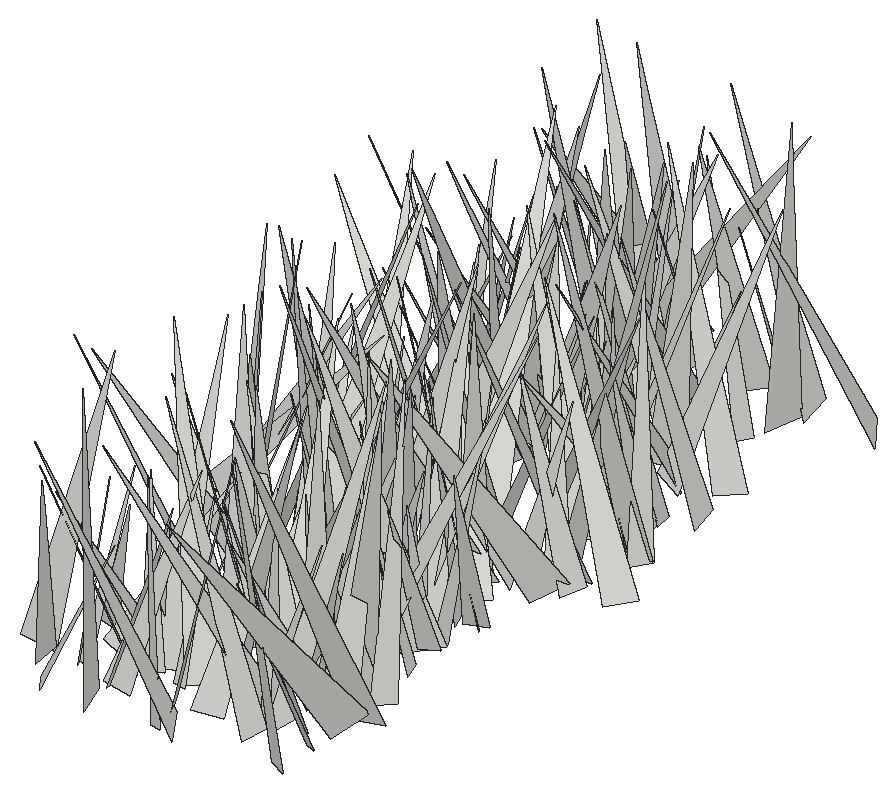
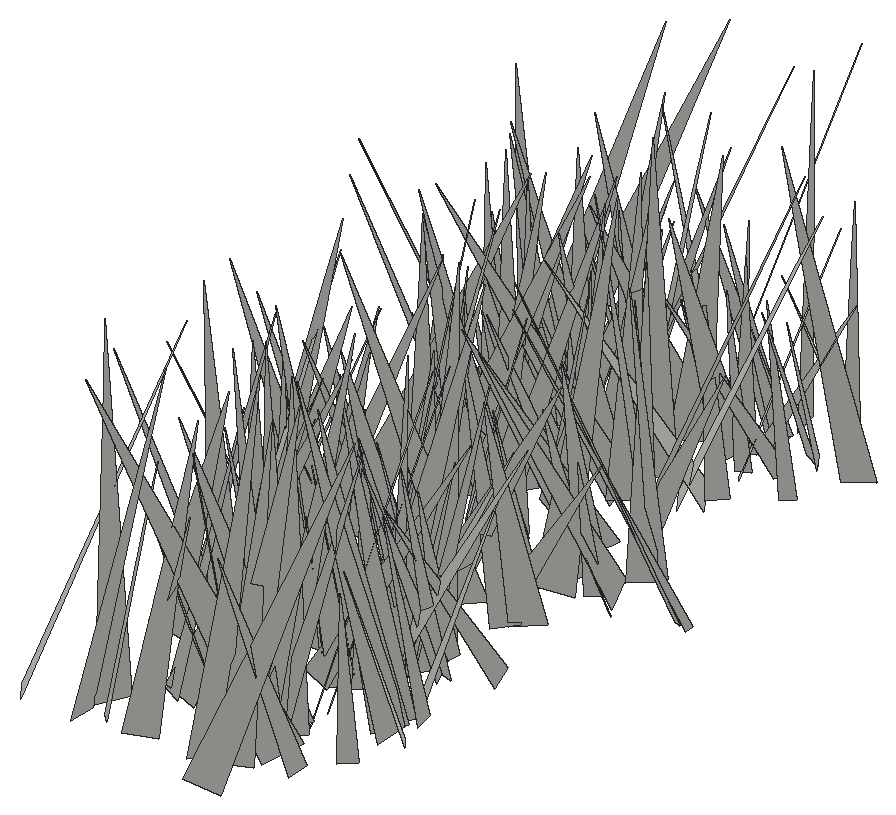
# SketchUp Ruby script. Lengths in inches.
U = 1.inch
M = Sketchup.active_model
def pt(a) = Geom::Point3d.new(a.map { |v| v * U })
def face(e, loops, mat)
  f = e.add_face(loops[0].map { |a| pt(a) })
  loops[1..].each { |l| e.add_face(l.map { |a| pt(a) }).erase! }
  f.material = f.back_material = mat if mat
  f
end
# faces: each face lists its corners as indices into pts; further lists are holes
def faces(e, pts, list, mat = nil) = list.each { |f| face(e, (f[0].is_a?(Array) ? f : [f]).map { |l| l.map { |i| pts[i] } }, mat) }
# xy, xz, yz: faces in a plane at the given z, y or x. An outline is a flat list of corners, or four numbers for a rectangle; further outlines are holes
def ring(l) = l.size == 4 ? [[l[0], l[1]], [l[2], l[1]], [l[2], l[3]], [l[0], l[3]]] : l.each_slice(2).to_a
def flat(e, list, mat, &to3) = list.each { |f| face(e, (f[0].is_a?(Array) ? f : [f]).map { |l| ring(l).map { |u, v| to3.(u, v) } }, mat) }
def xy(e, z, list, mat = nil) = flat(e, list, mat) { |x, y| [x, y, z] }
def xz(e, y, list, mat = nil) = flat(e, list, mat) { |x, z| [x, y, z] }
def yz(e, x, list, mat = nil) = flat(e, list, mat) { |y, z| [x, y, z] }
def lines(e, pts, list) = list.each { |a, b| e.add_line(pt(pts[a]), pt(pts[b])) }
# prism: a flat outline (further loops are holes) pulled along v
def prism(e, loops, v, mat = nil)
  f = face(e, loops, mat); d = Geom::Vector3d.new(v.map { |x| x * U })
  f.pushpull(f.normal.samedirection?(d) ? d.length : -d.length)
end
def box(e, o, s, mat = nil) = prism(e, [[o, [o[0] + s[0], o[1], o[2]], [o[0] + s[0], o[1] + s[1], o[2]], [o[0], o[1] + s[1], o[2]]]], [0, 0, s[2]], mat)
def at(x, y, z, deg = 0) = Geom::Transformation.translation(pt([x, y, z])) * Geom::Transformation.rotation(ORIGIN, Z_AXIS, deg.degrees)
def axes(o, x, y, z) = Geom::Transformation.new([*x, 0, *y, 0, *z, 0, *pt(o).to_a, 1])
def part(name) = M.definitions.add(name)
# library, detail: a bought-in or finely detailed component or shape, given as its bounding box
def library(name, o, s) = part(name).tap { |d| box(d.entities, o, s) }
def detail(e, o, s) = box(e.add_group.entities, o, s)
def put(e, d, t, mat = nil) = e.add_instance(d, t).tap { |i| i.material = mat if mat }
def group(e, t, mat = nil) = e.add_group.tap { |g| g.transformation = t; g.material = mat if mat }.entities
root = M.entities
c1 = part("fur_instance\#9")
p = [[0.8125,0,1.79],[0.67,-0.02,1.48],[0,-0.11,0],[0,0.11,0]]
faces(c1.entities,p,[[0,1,2,3]])
put(root,c1,axes([142.74,11.99,-27.1],[-6.5639,-4.29471,0.69968],[-4.06333,6.50273,1.7952],[1.55674,-1.13527,7.63588]))
put(root,c1,axes([138.88,11.62,-27.1],[6.72646,1.81373,2.96578],[2.30607,-7.16166,-0.85049],[-2.60144,-1.65881,6.91459]))
put(root,c1,axes([148.02,16.27,-27.1],[5.96387,-5.74764,0.45925],[-4.68382,-5.21453,-4.43673],[-3.36276,-2.93042,6.99418]))
put(root,c1,axes([135.31,13.3,-27.1],[5.21183,-0.69159,1.00189],[-0.40075,-5.13378,-1.45906],[-1.14955,-1.3458,5.051]))
put(root,c1,axes([136.49,11.45,-27.1],[3.11612,2.14822,0.04863],[2.13222,-3.08072,-0.53874],[0.26618,-0.47091,3.74631]))
put(root,c1,axes([147.85,11.98,-27.1],[-3.61019,-4.99925,2.09321],[-5.40705,3.49453,-0.97958],[0.37125,2.28107,6.08822]))
put(root,c1,axes([144.81,15.47,-27.1],[-6.99156,-3.62516,0.34789],[-3.32905,6.6672,2.57109],[1.47657,-2.13338,7.444]))
put(root,c1,axes([142.17,11.5,-27.1],[2.11114,4.26728,1.69749],[4.08085,-2.60007,1.46097],[-2.10662,-0.76029,4.53125]))
put(root,c1,axes([141.64,13.32,-27.1],[5.91305,2.63208,1.30513],[2.84881,-5.85376,-1.10147],[-0.71801,-1.54954,6.37799]))
put(root,c1,axes([147.875,14,-27.1],[-2.11494,-3.26023,0.3236],[-3.25153,2.04149,-0.68318],[-0.40176,0.64034,3.82562]))
put(root,c1,axes([138.71,13.3,-27.1],[4.6292,0.17151,0.50537],[0.17521,-4.6565,-0.02456],[-0.5041,-0.0434,4.63231]))
put(root,c1,axes([139.07,12.98,-27.1],[-0.2633,5.21725,2.01289],[5.21535,0.95622,-1.79623],[2.01778,-1.79073,4.90536]))
put(root,c1,axes([145.59,13.39,-27.1],[-7.05219,-0.0174,0.36445],[-0.04272,7.04446,-0.49029],[0.36236,0.49184,7.03515]))
put(root,c1,axes([138.22,16.61,-27.1],[-4.13321,-3.41194,0.20507],[-3.07913,3.85633,2.10107],[1.48403,-1.5014,4.93054]))
put(root,c1,axes([148.3125,16.93,-27.1],[0.33917,-8.30019,0.61155],[-8.21231,-0.43312,-1.32383],[-1.35096,0.54903,8.20095]))
put(root,c1,axes([138.89,14.33,-27.1],[-3.23089,-3.2407,0.20186],[-3.09319,2.98531,-1.58167],[-0.98745,1.25194,4.29408]))
put(root,c1,axes([134.44,13.88,-27.1],[1.86303,-6.4471,2.90273],[-6.99316,-1.23765,1.73947],[1.04242,3.21946,6.48153]))
put(root,c1,axes([146.71,14.99,-27.1],[-2.94659,-4.28728,0.79485],[-4.35538,2.84813,-0.78348],[-0.2081,1.09651,5.14289]))
put(root,c1,axes([136.61,13.6875,-27.1],[2.93854,2.24557,1.05284],[2.03507,-3.11619,0.96641],[-1.41759,0.18132,3.56983]))
put(root,c1,axes([145.97,14.85,-27.1],[-4.77809,0.40303,0.49366],[0.4272,4.79644,0.21897],[0.47289,-0.2608,4.79006]))
put(root,c1,axes([145.02,14.45,-27.1],[2.48119,3.58815,0.88423],[3.68479,-2.32113,-0.92071],[0.2811,-1.24521,4.2642]))
put(root,c1,axes([146.04,16.8,-27.1],[2.95419,-3.46444,1.08183],[-2.95275,-3.10527,-1.88109],[-2.11044,-0.50488,4.14621]))
put(root,c1,axes([139.31,14.87,-27.1],[1.67153,-3.68103,1.97281],[-4.08391,-1.88531,-0.05752],[-0.87388,1.76964,4.04237]))
put(root,c1,axes([136.89,13.69,-27.1],[1.45638,3.8911,0.37542],[3.87774,-1.48869,0.38679],[-0.49475,-0.21394,4.13668]))
put(root,c1,axes([138.44,16.03,-27.1],[0.50859,-3.54434,0.97529],[-3.61365,-0.30136,0.78924],[0.67458,1.05784,3.49258]))
put(root,c1,axes([135.71,16.69,-27.1],[0.50493,-3.90237,0.56248],[-3.75126,-0.30094,1.27958],[1.21364,0.69337,3.72104]))
put(root,c1,axes([142.125,16.17,-27.1],[6.74375,-1.56753,0.95704],[-1.61805,-6.79399,0.27364],[-0.86892,0.48558,6.91813]))
put(root,c1,axes([140.84,14.64,-27.1],[1.32341,3.79294,0.4756],[3.74321,-1.38791,0.65276],[-0.77522,-0.22654,3.9638]))
put(root,c1,axes([142.03,18.27,-27.1],[-4.79038,-5.44103,1.36632],[-5.2062,4.98101,1.5825],[2.08977,-0.06337,7.07448]))
put(root,c1,axes([144,16.3,-27.1],[0.99186,4.25892,2.03749],[4.71935,-0.95274,-0.30591],[-0.13232,-2.05608,4.36218]))
put(root,c1,axes([141.59,15.37,-27.1],[-4.74257,5.72398,1.5327],[5.90767,4.72004,0.65254],[0.46105,-1.60076,7.40474]))
put(root,c1,axes([143.11,13.57,-27.1],[-4.70627,4.28235,1.06672],[3.70191,4.67966,-2.45399],[2.40255,1.178,5.87073]))
put(root,c1,axes([136.97,15.39,-27.1],[0.32449,4.79651,0.65441],[4.29347,0.01783,-2.25961],[2.23626,-0.73022,4.24334]))
put(root,c1,axes([137.87,18.39,-27.1],[2.72527,-3.47225,0.02549],[-3.46346,-2.7159,0.33551],[0.24824,0.22715,4.40125]))
put(root,c1,axes([144.92,17.86,-27.1],[3.71508,-1.29272,0.27873],[-1.28155,-3.72443,-0.19222],[-0.32626,-0.0905,3.92887]))
put(root,c1,axes([145.99,19.27,-27.1],[2.29516,-7.21123,1.1617],[-7.23425,-2.07612,1.40519],[1.00849,1.5189,7.43607]))
put(root,c1,axes([139.01,19.41,-27.1],[-5.75391,-4.14909,0.07824],[-4.14913,5.75437,0.02082],[0.07564,0.02888,7.0938]))
put(root,c1,axes([139.53,15.29,-27.1],[-5.90287,3.96424,1.22936],[3.5461,5.92766,-2.08769],[2.15678,1.10365,6.7971]))
put(root,c1,axes([141.4,19.56,-27.1],[2.7716,-4.32676,0.73791],[-4.29866,-2.85215,-0.57784],[-0.88707,0.30254,5.10575]))
put(root,c1,axes([144.55,18.47,-27.1],[-1.98157,5.41612,3.08152],[6.10168,2.34277,-0.19399],[1.26474,-2.81671,5.76397]))
put(root,c1,axes([144.51,17.23,-27.1],[0.16131,6.95669,2.04491],[7.08472,0.28432,-1.5261],[1.54396,-2.03146,6.78915]))
put(root,c1,axes([146.39,17.65,-27.1],[-1.99924,6.11191,2.2816],[6.3463,2.375,-0.80119],[1.51181,-1.88733,6.38047]))
put(root,c1,axes([140.8,18.47,-27.1],[5.17413,-4.7343,3.23528],[-5.24163,-5.67192,0.08293],[-2.32507,2.25121,7.01272]))
put(root,c1,axes([143.2,18.56,-27.1],[-4.86777,3.35697,1.6535],[3.6105,4.92638,0.62739],[0.98366,-1.46972,5.8797]))
put(root,c1,axes([138.49,22.84,-27.1],[-6.95908,-3.88864,0.42907],[-3.38575,6.42493,3.31533],[1.96017,-2.70799,7.24975]))
put(root,c1,axes([140.65,20.63,-27.1],[4.51111,-4.76568,1.07484],[-4.75985,-4.61702,-0.49408],[-1.1004,0.43419,6.54353]))
put(root,c1,axes([143.24,20.07,-27.1],[3.93197,-0.07434,1.3447],[0.21137,-4.06439,-0.84276],[-1.33006,-0.86567,3.84131]))
put(root,c1,axes([146.99,18.65,-27.1],[-6.72767,0.28008,1.7782],[-0.11729,6.79671,-1.51427],[1.7963,1.49276,6.56102]))
put(root,c1,axes([143.32,19.18,-27.1],[3.71678,-0.58843,1.31141],[-0.99782,-3.67326,1.17982],[-1.0346,1.42876,3.57333]))
put(root,c1,axes([147.98,18.42,-27.1],[-6.09704,1.94582,1.05535],[1.61207,6.02238,-1.79053],[1.51697,1.42075,6.14444]))
put(root,c1,axes([147.14,21.22,-27.1],[-3.57828,-1.18752,0.86435],[-1.11493,3.67791,0.43741],[0.95617,-0.15551,3.74473]))
put(root,c1,axes([142.92,18.94,-27.1],[-3.90742,5.66938,0.63215],[5.60395,3.95813,-0.85923],[1.06639,-0.02677,6.83166]))
put(root,c1,axes([146.64,22.92,-27.1],[1.6071,-3.85332,0.26864],[-3.82652,-1.62792,-0.45895],[-0.52725,0.06941,4.14972]))
put(root,c1,axes([146.5625,22.87,-27.1],[1.94153,-7.03493,2.68991],[-6.84514,-2.80689,-2.40016],[-3.14163,1.7682,6.89195]))
put(root,c1,axes([138.73,21.43,-27.1],[-2.74524,3.88345,0.46197],[3.73915,2.44095,1.70042],[-1.14601,-1.33847,4.4414]))
put(root,c1,axes([138.39,18.46,-27.1],[6.17595,4.1917,0.11311],[3.92557,-5.85042,2.46738],[-1.47413,1.98185,7.04448]))
put(root,c1,axes([145.65,22.14,-27.1],[-2.59622,-3.87524,1.56211],[-4.17566,2.47102,-0.8099],[0.14666,1.75346,4.59368]))
put(root,c1,axes([142.77,21.34,-27.1],[4.39475,-2.24157,1.41228],[-2.61052,-4.13054,1.56743],[-0.4521,2.06082,4.67778]))
put(root,c1,axes([146.18,23.16,-27.1],[2.32734,-2.83374,0.7234],[-2.82694,-2.41664,-0.37171],[-0.74954,0.31569,3.64807]))
put(root,c1,axes([142.69,22.97,-27.1],[-2.18314,-4.32344,1.23175],[-4.48368,1.99494,-0.94459],[-0.32548,1.51774,4.75036]))
put(root,c1,axes([143.6875,24.62,-27.1],[-2.92587,-7.18113,1.16279],[-7.26033,2.80394,-0.95233],[-0.45638,1.43204,7.69561]))
put(root,c1,axes([144.07,20.84,-27.1],[-6.55777,-1.69063,0.96933],[-1.94723,5.82112,-3.02077],[0.07829,3.17151,6.06115]))
put(root,c1,axes([143.35,25.17,-27.1],[6.03142,-3.81553,0.06105],[-3.78285,-5.99326,-0.84318],[-0.50203,-0.68018,7.08699]))
put(root,c1,axes([141.83,22.16,-27.1],[3.01287,6.59159,3.14785],[6.68601,-3.85992,1.68335],[-2.94198,-2.02171,7.04931]))
put(root,c1,axes([141.3,20.08,-27.1],[8.13391,1.72844,0.70897],[1.41113,-7.75982,2.72846],[-1.22428,2.53935,7.85515]))
put(root,c1,axes([144.98,21.31,-27.1],[4.52009,6.67395,0.30614],[6.59904,-4.40227,-1.46264],[1.04307,-1.07006,7.92676]))
put(root,c1,axes([142.47,25.44,-27.1],[1.32188,-7.44707,0.58602],[-7.30684,-1.16527,1.67389],[1.55318,0.85612,7.37593]))
put(root,c1,axes([136.04,25.33,-27.1],[5.72206,-2.67718,0.30846],[-2.55509,-5.6197,-1.37653],[-0.85672,-1.12072,6.16558]))
put(root,c1,axes([137.13,23.32,-27.1],[6.97385,3.06548,2.09729],[3.25235,-7.19468,-0.2986],[-1.79388,-1.12684,7.61201]))
put(root,c1,axes([137.36,22.89,-27.1],[3.68214,4.39884,2.0354],[4.4735,-4.06815,0.69917],[-1.86561,-1.07294,5.69378]))
put(root,c1,axes([143.95,25.19,-27.1],[-6.33507,2.2676,3.27677],[3.13305,6.63723,1.4641],[2.46237,-2.61105,6.56746]))
put(root,c1,axes([142.98,24.62,-27.1],[2.13927,-3.81253,0.27989],[-3.71667,-1.99926,1.17453],[0.89447,0.81104,4.21098]))
put(root,c1,axes([146.87,25.55,-27.1],[2.00782,-4.43373,0.05819],[-4.43409,-2.00742,0.0429],[0.01508,0.0707,4.86698]))
put(root,c1,axes([144.14,22.46,-27.1],[-3.10832,3.75001,0.92239],[3.63037,3.24121,-0.94342],[1.31674,-0.08395,4.77852]))
put(root,c1,axes([141.85,22.47,-27.1],[4.95008,1.27612,1.12304],[0.89586,-4.89693,1.61571],[-1.4447,1.33589,4.84988]))
put(root,c1,axes([145.67,23.41,-27.1],[1.56469,4.5597,1.40699],[4.65343,-1.78584,0.61247],[-1.05645,-1.11294,4.78163]))
put(root,c1,axes([146.74,23.44,-27.1],[-4.01234,0.85775,1.7856],[0.34464,4.27421,-1.27879],[1.95072,1.00913,3.89863]))
put(root,c1,axes([144.87,28.2,-27.1],[1.87232,-8.06563,0.81969],[-7.60481,-2.03883,-2.69107],[-2.80947,0.14362,7.83059]))
put(root,c1,axes([146.05,25.52,-27.1],[4.40996,1.53054,2.75088],[1.88618,-5.07543,-0.19988],[-2.52036,-1.1203,4.66373]))
put(root,c1,axes([136.17,24.15,-27.1],[2.58836,6.22661,1.98748],[6.38761,-2.86286,0.6503],[-1.38536,-1.56644,6.71174]))
put(root,c1,axes([147.49,29.34,-27.1],[4.76692,-6.38187,0.99404],[-5.33821,-4.5884,-3.85875],[-3.63592,-1.6304,6.96863]))
put(root,c1,axes([146.85,25.67,-27.1],[-5.72763,-4.55632,1.57593],[-4.80185,5.61014,-1.23206],[0.43111,1.95337,7.21442]))
put(root,c1,axes([144.26,24.51,-27.1],[3.571,6.90444,0.98118],[6.89309,-3.32732,-1.67343],[1.05801,-1.62595,7.59098]))
put(root,c1,axes([138.26,28.04,-27.1],[1.76512,-7.95634,1.31885],[-8.03843,-1.84494,-0.37166],[-0.65291,1.20466,8.14131]))
put(root,c1,axes([145.48,23.91,-27.1],[5.43527,-3.00495,4.38513],[-4.48513,-5.95873,1.47596],[-2.85354,3.64214,6.0327]))
put(root,c1,axes([142.23,25.63,-27.1],[0.54119,7.40359,2.44886],[7.61955,0.0202,-1.74498],[1.65906,-2.50787,7.21533]))
put(root,c1,axes([132.29,27.08,-27.1],[4.7067,5.43888,0.18038],[4.50837,-3.76361,-4.15655],[3.04771,-2.83211,5.87006]))
put(root,c1,axes([145.35,26.72,-27.1],[-4.286,2.05614,0.85108],[2.13965,4.31523,0.34994],[0.6115,-0.68765,4.74078]))
put(root,c1,axes([132.9375,27,-27.1],[5.32286,5.30667,0.20638],[4.93366,-4.8331,-2.97258],[1.96528,-2.23975,6.90343]))
put(root,c1,axes([138.51,25.88,-27.1],[-1.52341,4.48001,0.30788],[4.47725,1.54034,-0.26007],[0.34571,-0.20714,4.72479]))
put(root,c1,axes([145.82,29.09,-27.1],[-3.34335,-1.51871,0.13226],[-1.40215,3.18862,1.16988],[0.59829,-1.01398,3.48078]))
put(root,c1,axes([144.09,28.92,-27.1],[1.85268,-6.56464,1.39244],[-6.70428,-1.74747,0.68181],[0.2934,1.52239,6.78691]))
put(root,c1,axes([138.0625,25.94,-27.1],[-5.38629,2.97439,0.98855],[2.72826,5.41671,-1.43257],[1.54299,0.80541,5.98388]))
put(root,c1,axes([135.36,28.14,-27.1],[3.3764,2.66955,0.1135],[2.47122,-3.05035,-1.76859],[1.01611,-1.452,3.92412]))
put(root,c1,axes([136.83,27.32,-27.1],[-1.83169,3.1238,0.57494],[3.14275,1.87858,-0.19441],[0.4602,-0.39568,3.61599]))
put(root,c1,axes([140.72,26.51,-27.1],[1.48106,4.37962,0.44895],[4.22706,-1.54701,1.14671],[-1.23071,-0.04293,4.4788]))
put(root,c1,axes([143.94,30.95,-27.1],[-6.24986,-4.52728,1.84324],[-4.17742,6.50052,1.80193],[2.5383,-0.44892,7.504]))
put(root,c1,axes([145.62,27.11,-27.1],[-3.60755,4.52257,0.00535],[4.517,3.60276,0.29145],[-0.22451,-0.18592,5.77782]))
put(root,c1,axes([138.86,24.49,-27.1],[-6.04626,5.73242,0.3376],[5.11125,5.59588,-3.47751],[2.61721,2.31459,7.57131]))
put(root,c1,axes([148.16,29.96,-27.1],[-4.52682,2.09063,1.69581],[2.46981,4.54531,0.98938],[1.07078,-1.64562,4.88712]))
put(root,c1,axes([139.35,29.24,-27.1],[-2.95637,3.32548,0.26078],[3.10336,2.61427,1.84435],[-1.22309,-1.40488,4.04936]))
put(root,c1,axes([146,29.38,-27.1],[1.71183,-4.04593,1.56999],[-4.29437,-1.33542,1.2409],[0.62675,1.9005,4.21427]))
put(root,c1,axes([147.77,30.9375,-27.1],[-2.28095,-6.51713,0.89519],[-6.46928,2.05047,-1.55597],[-1.19279,1.34151,6.72716]))
put(root,c1,axes([144.45,27.84,-27.1],[1.52611,3.71718,0.33458],[3.41655,-1.5369,1.49113],[-1.50217,0.28087,3.73135]))
put(root,c1,axes([136.18,26.61,-27.1],[6.68377,2.4417,1.0502],[1.89436,-6.36953,2.75283],[-1.86446,2.28139,6.56175]))
put(root,c1,axes([141.28,31.02,-27.1],[-4.99483,-3.69291,1.05885],[-3.66459,5.10128,0.50484],[1.15306,0.21561,6.19121]))
put(root,c1,axes([137.96,31.39,-27.1],[3.51302,-4.23345,1.0034],[-4.35037,-3.40123,0.88101],[0.05668,1.33409,5.43021]))
put(root,c1,axes([150.14,30.4,-27.1],[-3.49983,5.63032,0.78088],[5.54982,3.18646,1.89866],[-1.22869,-1.64469,6.35172]))
put(root,c1,axes([139.46,33.86,-27.1],[4.72004,-5.82808,0.22381],[-5.80637,-4.72269,-0.52693],[-0.55017,-0.15829,7.48115]))
put(root,c1,axes([140.2,30.79,-27.1],[-0.29437,7.39176,2.68978],[7.28817,1.26884,-2.68928],[2.95898,-2.3899,6.89148]))
put(root,c1,axes([141.62,30.83,-27.1],[-4.54084,5.90887,0.08971],[5.53212,4.21055,2.68494],[-2.07809,-1.7025,6.95162]))
put(root,c1,axes([146.15,31.51,-27.1],[-2.40866,3.6867,1.3913],[3.88066,2.50239,0.08743],[0.68406,-1.21467,4.40293]))
put(root,c1,axes([143.33,30.94,-27.1],[5.62442,0.34622,0.61815],[0.22701,-5.5658,1.05184],[-0.67115,1.01884,5.53603]))
put(root,c1,axes([147,36.17,-27.1],[-5.34969,-3.46152,0.37635],[-2.75195,4.62606,3.43064],[2.1332,-2.713,5.36954]))
put(root,c1,axes([148.27,33.78,-27.1],[-1.48143,-7.59825,2.03928],[-7.84224,1.26126,-0.99758],[-0.62555,2.18232,7.67677]))
put(root,c1,axes([144.22,32.82,-27.1],[6.32443,-0.86949,0.03215],[-0.87008,-6.31952,0.24926],[0.00213,0.25131,6.37905]))
put(root,c1,axes([137.33,30.75,-27.1],[-3.85678,5.81728,0.33644],[5.7739,3.8696,-0.71896],[0.78484,0.11882,6.94252]))
put(root,c1,axes([140.49,33.93,-27.1],[-3.6362,-3.51378,0.23491],[-3.4583,3.49912,-1.19165],[-0.6648,1.01649,4.91412]))
put(root,c1,axes([146.64,31.56,-27.1],[-7.17026,0.40545,3.85637],[-0.86926,7.73252,-2.42922],[3.77894,2.54801,6.75839]))
put(root,c1,axes([147.41,35.46,-27.1],[4.28198,-1.79299,1.3249],[-1.43721,-4.41332,-1.32759],[-1.70429,-0.78312,4.44833]))
put(root,c1,axes([147.49,34.14,-27.1],[-3.51582,-2.14374,0.80605],[-2.26912,3.46073,-0.69338],[0.31056,1.01688,4.05904]))
put(root,c1,axes([145.63,33.25,-27.1],[-2.86561,6.0597,1.12131],[6.09085,2.59686,1.53195],[-0.93747,-1.65086,6.5257]))
put(root,c1,axes([146.14,35.09,-27.1],[-0.76363,-5.08076,1.72351],[-5.30047,0.98391,0.55201],[0.83046,1.60796,5.10809]))
put(root,c1,axes([148.84,33.27,-27.1],[-5.6137,1.8249,1.28834],[1.63706,5.7317,-0.98561],[1.51991,0.56669,5.82001]))
put(root,c1,axes([139.04,38.04,-27.1],[0.62863,-8.27068,0.12443],[-8.26435,-0.63324,-0.33804],[-0.34653,0.09834,8.28764]))
put(root,c1,axes([139.91,36.49,-27.1],[2.79879,-2.29313,0.37979],[-2.08936,-2.74248,-1.16161],[-1.01846,-0.6755,3.42672]))
put(root,c1,axes([143.89,34.13,-27.1],[3.61402,1.40651,0.81578],[1.29809,-3.69316,0.61679],[-0.97915,0.29527,3.8287]))
put(root,c1,axes([145.46,39.77,-27.1],[-5.2335,-6.40482,0.23356],[-5.52847,4.66397,4.0186],[3.24225,-2.38569,7.22925]))
put(root,c1,axes([138.54,35.79,-27.1],[-6.31827,-0.38458,1.65434],[-0.20418,6.49842,0.73085],[1.68614,-0.65417,6.28763]))
put(root,c1,axes([139.84,33.81,-27.1],[4.20978,2.5999,1.29958],[2.36123,-4.39284,1.13935],[-1.69498,0.33775,4.81493]))
put(root,c1,axes([138.58,36.76,-27.1],[-1.9531,-3.93926,0.49775],[-3.87343,2.01224,0.72636],[0.87298,0.11511,4.33645]))
put(root,c1,axes([144.86,35.36,-27.1],[-0.32853,3.96848,1.56907],[4.26678,0.33258,0.05223],[0.07349,-1.56822,3.98171]))
put(root,c1,axes([138.9,37.02,-27.1],[-1.97091,-5.99186,1.73382],[-5.97714,2.33419,1.27215],[1.7839,1.20092,6.17807]))
put(root,c1,axes([141.57,32.63,-27.1],[-2.88963,7.72101,0.14725],[7.7077,2.8933,-0.45358],[0.4764,0.02131,8.23153]))
put(root,c1,axes([138.07,34.8,-27.1],[3.76541,-0.98312,2.37268],[-1.72485,-4.08783,1.04352],[-1.9029,1.75998,3.74912]))
put(root,c1,axes([141.42,34.72,-27.1],[3.44436,3.22324,0.28553],[3.18394,-3.45028,0.54084],[-0.57733,0.20181,4.68619]))
put(root,c1,axes([148.54,37.59,-27.1],[-6.39849,-1.36399,1.46981],[-1.16574,6.52941,0.98452],[1.63152,-0.68393,6.46776]))
put(root,c1,axes([136.5,38.5625,-27.1],[-3.05725,-3.63504,0.09512],[-3.51202,2.98398,1.15363],[0.94245,-0.67208,4.60753]))
put(root,c1,axes([135.56,34.65,-27.1],[4.79921,1.03907,0.41248],[0.79797,-4.45725,1.94381],[-0.78297,1.82633,4.50929]))
put(root,c1,axes([138.25,36.11,-27.1],[-2.58112,4.19595,2.18678],[4.13957,3.20902,-1.27135],[2.29171,-1.07069,4.75939]))
put(root,c1,axes([139.25,37.22,-27.1],[-5.24888,-4.54366,0.15791],[-4.36596,4.97023,-2.11085],[-1.26815,1.69482,6.61361]))
put(root,c1,axes([147.39,36.5,-27.1],[-6.20853,-2.44848,0.56631],[-2.51301,6.03462,-1.45936],[-0.02325,1.56521,6.51238]))
put(root,c1,axes([139.16,38.56,-27.1],[4.92449,-2.5321,0.51516],[-2.43841,-4.92066,-0.87679],[-0.85503,-0.55051,5.46748]))
put(root,c1,axes([141.125,39.2,-27.1],[-0.84326,-5.89202,0.02664],[-5.53518,0.78295,-2.04363],[-2.01949,0.3143,5.59022]))
put(root,c1,axes([145.51,34.77,-27.1],[4.61833,5.37447,0.17353],[5.34108,-4.61135,0.67253],[-0.62281,0.30742,7.05419]))
put(root,c1,axes([139.85,38.79,-27.1],[2.97269,-7.01093,0.81561],[-6.80259,-2.60982,2.35986],[1.88234,1.64042,7.24024]))
put(root,c1,axes([137.6,35.75,-27.1],[5.0446,1.96996,1.21492],[1.59207,-5.06819,1.60732],[-1.6799,1.1124,5.17158]))
put(root,c1,axes([137.68,35.8,-27.1],[0.92539,5.82013,0.73982],[5.78512,-1.02986,0.86568],[-0.97656,-0.58571,5.82931]))
put(root,c1,axes([140.22,37.95,-27.1],[3.37975,2.64749,1.02841],[2.82915,-3.2791,-0.85611],[-0.25046,-1.31446,4.20701]))
put(root,c1,axes([136.41,39.77,-27.1],[0.97454,-6.53217,0.4424],[-5.83998,-0.6651,3.04417],[2.95966,0.83851,5.86106]))
put(root,c1,axes([139.24,40.72,-27.1],[-5.93761,-4.29126,0.84113],[-3.95201,5.87307,2.0655],[1.8719,-1.21235,7.02879]))
put(root,c1,axes([142.92,37.33,-27.1],[-0.41482,4.98169,1.32883],[5.15587,0.40286,0.09923],[0.00793,-1.33251,4.99795]))
put(root,c1,axes([138.95,42.25,-27.1],[-5.78164,-4.6449,0.78576],[-4.06196,5.54542,2.89287],[2.386,-1.8147,6.82889]))
put(root,c1,axes([144.78,40.01,-27.1],[2.7668,-7.06079,2.0724],[-7.35623,-2.5972,0.97226],[0.18857,2.28135,7.52095]))
put(root,c1,axes([135.76,39.21,-27.1],[4.33952,0.70183,1.00017],[0.70812,-4.45199,0.05164],[-0.99573,-0.10739,4.3956]))
put(root,c1,axes([144.18,38.46,-27.1],[2.59525,5.12132,1.23508],[5.09738,-2.78884,0.85303],[-1.33041,-0.69505,5.67763]))
put(root,c1,axes([141.72,38.09,-27.1],[2.74983,3.97442,1.3241],[3.39736,-3.04242,2.07665],[-2.45097,0.24187,4.36407]))
put(root,c1,axes([145.03,40.47,-27.1],[-6.53044,0.59698,0.86107],[0.69842,6.53195,0.76827],[0.78105,-0.84949,6.51251]))
put(root,c1,axes([145.6875,38.91,-27.1],[2.61038,6.20008,1.07332],[6.21386,-2.35716,-1.49626],[0.99041,-1.55238,6.55868]))
put(root,c1,axes([141,41.61,-27.1],[-1.51779,-7.89387,2.17922],[-8.18213,1.37007,-0.73587],[-0.33897,2.275,8.00471]))
put(root,c1,axes([136.43,40.5,-27.1],[4.89354,-4.52263,1.72188],[-4.82903,-4.72322,1.31813],[-0.31551,2.14541,6.53173]))
put(root,c1,axes([144.41,43.53,-27.1],[-1.51333,-7.7582,0.0595],[-7.60064,1.47034,-1.59746],[-1.5568,0.36304,7.74132]))
put(root,c1,axes([148.1,39.79,-27.1],[-2.07893,6.71015,1.41675],[6.64432,1.60395,2.15305],[-1.69892,-1.93817,6.68674]))
put(root,c1,axes([139.9,43.09,-27.1],[6.8807,-3.2851,0.24825],[-3.20439,-6.80705,-1.26238],[-0.76512,-1.03432,7.51946]))
put(root,c1,axes([136.06,40.77,-27.1],[7.69259,-0.4984,1.40276],[-0.64413,-7.77059,0.77146],[-1.3421,0.87272,7.67002]))
put(root,c1,axes([135.27,41,-27.1],[2.99336,2.37967,0.42143],[2.41657,-2.95437,-0.48225],[-0.02533,-0.63994,3.79348]))
put(root,c1,axes([139.2,43.29,-27.1],[5.34448,-4.72432,0.68412],[-4.69665,-5.3877,-0.51471],[-0.85369,0.0645,7.11462]))
put(root,c1,axes([144.73,43.62,-27.1],[-3.08937,-5.14938,0.76665],[-5.09175,3.1744,0.80332],[1.08532,0.23487,5.95105]))
put(root,c1,axes([139.33,44.3,-27.1],[-0.1774,-7.7519,1.13116],[-7.17611,0.61466,3.08685],[3.14245,0.96602,7.113]))
put(root,c1,axes([139.78,43.24,-27.1],[-2.67742,-5.68655,1.10676],[-5.79247,2.6077,-0.61446],[-0.09527,1.2623,6.25523]))
put(root,c1,axes([139.37,42.57,-27.1],[3.36914,-5.54095,2.01408],[-5.73384,-2.5398,2.60427],[1.37175,2.99283,5.93894]))
put(root,c1,axes([143.16,42.86,-27.1],[2.4928,2.63766,0.46244],[2.65596,-2.35455,-0.88721],[0.34203,-0.94022,3.51911]))
put(root,c1,axes([140.04,43.83,-27.1],[0.54062,-3.9189,1.26852],[-4.01221,-0.79056,-0.73238],[-0.93225,1.12979,3.88763]))
put(root,c1,axes([136.01,43.625,-27.1],[-2.23187,2.81976,1.51549],[3.01775,2.4697,-0.15093],[1.06816,-1.08561,3.59298]))
put(root,c1,axes([141.62,43.41,-27.1],[-4.16616,6.68617,2.08588],[7.00105,3.90518,1.46546],[-0.20279,-2.54114,7.74043]))
put(root,c1,axes([149.46,47.09,-27.1],[-6.65977,-5.09555,0.25994],[-4.96209,6.56797,1.61994],[1.1874,-1.13219,8.22757]))
put(root,c1,axes([139.34,46.49,-27.1],[3.47226,-5.91321,0.27335],[-5.89868,-3.48291,-0.41506],[-0.49636,0.02495,6.84473]))
put(root,c1,axes([146.22,45.4,-27.1],[7.26083,-2.43104,1.92439],[-2.31077,-7.51014,-0.76873],[-2.06726,-0.14373,7.61831]))
put(root,c1,axes([140.98,43.96,-27.1],[-3.67972,-3.6806,3.42599],[-4.33109,4.47676,0.15761],[2.55458,2.28831,5.20214]))
put(root,c1,axes([139.25,48.64,-27.1],[4.10096,-6.21113,0.1393],[-5.64172,-3.79303,-3.03306],[-2.60165,-1.56533,6.79681]))
put(root,c1,axes([138.4375,44.63,-27.1],[5.80573,-6.03364,0.3689],[-5.4436,-4.99608,3.95649],[2.62833,2.98023,7.37953]))
put(root,c1,axes([145.56,46.7,-27.1],[-3.59225,-3.71334,1.0598],[-3.39845,3.72735,1.54069],[1.83374,-0.36648,4.93148]))
put(root,c1,axes([145.77,43.52,-27.1],[-5.65883,0.17912,0.29432],[0.09895,5.4838,-1.43499],[0.33003,1.4272,5.47679]))
put(root,c1,axes([140.63,46.625,-27.1],[6.98287,-2.99298,2.96369],[-2.61118,-7.57832,-1.50091],[-3.30502,-0.33623,7.44753]))
put(root,c1,axes([143.66,46.95,-27.1],[3.60817,-5.34608,1.25489],[-5.24687,-3.79935,-1.09972],[-1.62036,0.39817,6.35531]))
put(root,c1,axes([137.07,45.37,-27.1],[4.6922,-0.3007,0.23761],[-0.32477,-4.66947,0.50417],[-0.20347,0.51889,4.67471]))
put(root,c1,axes([146.5,47.02,-27.1],[-7.391,-1.41623,2.02124],[-1.14457,7.62073,1.15434],[2.18657,-0.79801,7.4364]))
